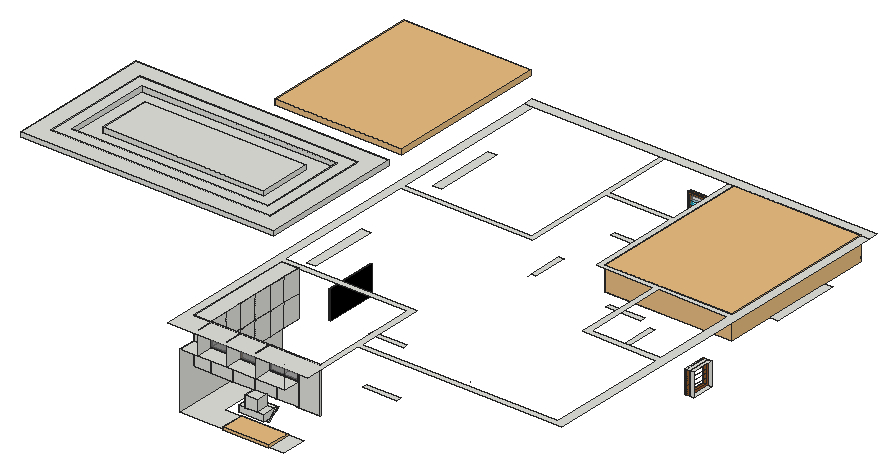
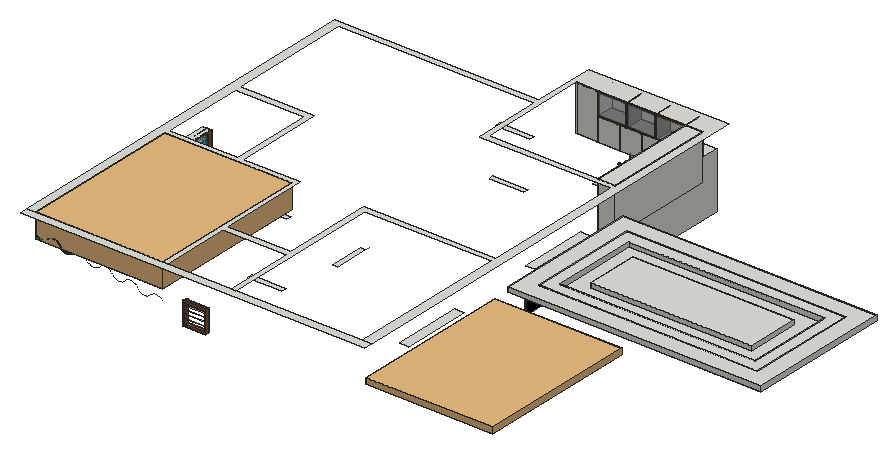
# SketchUp Ruby script. Lengths in inches.
U = 1.inch
M = Sketchup.active_model
def pt(a) = Geom::Point3d.new(a.map { |v| v * U })
def face(e, loops, mat)
  f = e.add_face(loops[0].map { |a| pt(a) })
  loops[1..].each { |l| e.add_face(l.map { |a| pt(a) }).erase! }
  f.material = f.back_material = mat if mat
  f
end
# faces: each face lists its corners as indices into pts; further lists are holes
def faces(e, pts, list, mat = nil) = list.each { |f| face(e, (f[0].is_a?(Array) ? f : [f]).map { |l| l.map { |i| pts[i] } }, mat) }
# xy, xz, yz: faces in a plane at the given z, y or x. An outline is a flat list of corners, or four numbers for a rectangle; further outlines are holes
def ring(l) = l.size == 4 ? [[l[0], l[1]], [l[2], l[1]], [l[2], l[3]], [l[0], l[3]]] : l.each_slice(2).to_a
def flat(e, list, mat, &to3) = list.each { |f| face(e, (f[0].is_a?(Array) ? f : [f]).map { |l| ring(l).map { |u, v| to3.(u, v) } }, mat) }
def xy(e, z, list, mat = nil) = flat(e, list, mat) { |x, y| [x, y, z] }
def xz(e, y, list, mat = nil) = flat(e, list, mat) { |x, z| [x, y, z] }
def yz(e, x, list, mat = nil) = flat(e, list, mat) { |y, z| [x, y, z] }
def lines(e, pts, list) = list.each { |a, b| e.add_line(pt(pts[a]), pt(pts[b])) }
# prism: a flat outline (further loops are holes) pulled along v
def prism(e, loops, v, mat = nil)
  f = face(e, loops, mat); d = Geom::Vector3d.new(v.map { |x| x * U })
  f.pushpull(f.normal.samedirection?(d) ? d.length : -d.length)
end
def box(e, o, s, mat = nil) = prism(e, [[o, [o[0] + s[0], o[1], o[2]], [o[0] + s[0], o[1] + s[1], o[2]], [o[0], o[1] + s[1], o[2]]]], [0, 0, s[2]], mat)
def at(x, y, z, deg = 0) = Geom::Transformation.translation(pt([x, y, z])) * Geom::Transformation.rotation(ORIGIN, Z_AXIS, deg.degrees)
def axes(o, x, y, z) = Geom::Transformation.new([*x, 0, *y, 0, *z, 0, *pt(o).to_a, 1])
def part(name) = M.definitions.add(name)
# library, detail: a bought-in or finely detailed component or shape, given as its bounding box
def library(name, o, s) = part(name).tap { |d| box(d.entities, o, s) }
def detail(e, o, s) = box(e.add_group.entities, o, s)
def put(e, d, t, mat = nil) = e.add_instance(d, t).tap { |i| i.material = mat if mat }
def group(e, t, mat = nil) = e.add_group.tap { |g| g.transformation = t; g.material = mat if mat }.entities
root = M.entities
M.materials.add("[Color C08]").color = [102, 51, 0]
M.materials.add("[Color_009]").color = [0, 0, 0]
M.materials.add("[Translucent Glass Gray]").color = [128, 128, 128]
M.materials["[Translucent Glass Gray]"].alpha = 0.5
M.materials.add("[Translucent Glass Tinted]1").color = [7, 201, 240]
M.materials["[Translucent Glass Tinted]1"].alpha = 0.48
M.materials.add("[Translucent_Glass_Gray]3").color = [128, 128, 128]
M.materials["[Translucent_Glass_Gray]3"].alpha = 0.5
M.materials.add("[Wood Cherry Original]").color = [152, 86, 42]
M.materials.add("[Wood Floor Parquet]").color = [145, 89, 39]
c1 = library("Gas cooktop",[0,0,34.52],[24.41,48.07,2.63])
c2 = part("Inclined chimney")
g1 = group(c2.entities,at(1.97,2.08,2.89))
xy(g1,0,[[0,7.9,31.3,13.68]])
xy(g1,11.29,[[0,0,31.3,13.68]])
xz(g1,13.68,[[0,0,31.3,11.29]])
yz(g1,0,[[7.9,0,0,11.29,13.68,11.29,13.68,0]])
yz(g1,31.3,[[7.9,0,13.68,0,13.68,11.29,0,11.29]])
g2 = group(c2.entities,at(0,9.85,0.4))
g3 = group(g2,at(0,0.61,0.43))
prism(g3,[[[35.24,0,0],[35.24,-3.39,4.84],[35.24,-3.58,4.7],[35.24,-0.29,0]]],[-35.24,0,0])
g4 = group(g2,at(0,-3.21,4.99))
prism(g4,[[[35.24,-0.2,-0.12],[35.24,-3.16,5],[0,-3.16,5],[0,-0.2,-0.12]]],[0,0.2,0.12])
g5 = group(g2,at(0,-6.27,10.27))
prism(g5,[[[35.24,-0.19,-0.14],[35.24,-3.58,4.7],[0,-3.58,4.7],[0,-0.19,-0.14]]],[0,0.19,0.14])
g6 = group(g2,at(0,0.61,0.43))
prism(g6,[[[35.24,0,0],[35.24,0.96,0],[35.24,-9.52,14.96],[35.24,-10.16,14.51]]],[-35.24,0,0])
g7 = group(c2.entities,at(10.24,3.95,20.8))
box(g7,[0,0,-6.62],[14.76,11.8125,20.56])
g8 = group(c2.entities,at(0,10.1,0))
prism(g8,[[[35.24,0.46,0],[35.24,1.33,0],[35.24,1.33,0.83],[35.24,1.01,0.83],[35.24,0.37,0.83],[35.24,0,0.83],[35.24,0,0.64]]],[-35.24,0,0])
c3 = part("Inclined+chimney")
put(c3.entities,c2,at(34.17,38.97,0.69))
c4 = part("ventilator")
g9 = group(c4.entities,at(0,0,0))
xy(g9,0,[[0,0,24,1],[0,1,24,6.83]],"[Wood Floor Parquet]")
xy(g9,1.75,[[2,0,22,6.83]],"[Wood Floor Parquet]")
xy(g9,21.87,[[2,0,22,6.83]],"[Wood Cherry Original]")
xy(g9,23.62,[[0,0,24,1],[0,1,24,6.83]],"[Wood Floor Parquet]")
xz(g9,0,[[[0,0,24,23.62],[2,1.75,22,21.87]]],"[Wood Floor Parquet]")
xz(g9,6.83,[[[0,0,24,23.62],[2,1.75,22,21.87]]],"[Wood Cherry Original]")
yz(g9,0,[[0,0,1,23.62],[1,0,6.83,23.62]],"[Wood Floor Parquet]")
yz(g9,2,[[0,1.75,6.83,1.75,6.83,7.66,0,3.5],[0,3.5,6.83,7.66,6.83,11.8125,0,7.66],[0,7.66,6.83,11.8125,6.83,15.97,0,11.8125],[0,11.8125,6.83,15.97,6.83,20.12,0,15.97],[0,15.97,6.83,20.12,6.83,21.87,0,21.87]],"[Wood Floor Parquet]")
yz(g9,22,[[0,1.75,0,3.5,6.83,7.66,6.83,1.75],[0,3.5,0,7.66,6.83,11.8125,6.83,7.66],[0,7.66,0,11.8125,6.83,15.97,6.83,11.8125],[0,11.8125,0,15.97,6.83,20.12,6.83,15.97],[0,15.97,0,21.87,6.83,21.87,6.83,20.12]],"[Wood Floor Parquet]")
yz(g9,24,[[0,0,1,23.62],[1,0,6.83,23.62]],"[Wood Floor Parquet]")
p = [[2,0,3.5],[2,6.83,7.66],[22,6.83,7.66],[22,0,3.5],[2,6.83,11.8125],[2,0,7.66],
  [22,0,7.66],[22,6.83,11.8125],[2,0,11.8125],[2,6.83,15.97],[22,6.83,15.97],[22,0,11.8125],
  [2,6.83,20.12],[2,0,15.97],[22,0,15.97],[22,6.83,20.12]]
faces(g9,p,[[0,1,2,3],[4,5,6,7],[8,9,10,11]],"[Translucent Glass Tinted]1")
faces(g9,p,[[12,13,14,15]],"[Translucent Glass Gray]")
c5 = library("Group\#27",[0,0,0],[132.5,168.5,25.21])
c6 = part("Component\#5")
box(c6.entities,[0,0,0],[30.3,0.18,23.6])
c7 = part("Group\#29")
xy(c7.entities,23.6,[[0,0.18,30.3,0.28]])
xz(c7.entities,0.28,[[[0,0,30.3,23.6],[1,1,29.3,22.6]]],"[Color C08]")
put(c7.entities,c6,at(0,0,0),"[Translucent_Glass_Gray]3")
c8 = library("Group\#16",[0,0,0],[132.5,168.5,6])
xy(root,37,[[301.397,9,409.897,9,409.897,35,327.397,35,327.397,141.5,301.397,141.5]])
xy(root,72,[[301.397,27,319.217,141.5],[643.397,241.399,652.397,265.051]])
xy(root,72.2,[[319.597,26.82,342.097,27],[342.497,26.82,364.997,27],[365.397,26.82,387.897,27],[388.297,26.82,410.797,27],[411.197,26.82,433.697,27],
  [319.217,27.2,319.397,45.883],[319.217,46.283,319.397,64.967],[319.217,65.367,319.397,84.05],[319.217,84.45,319.397,103.133],[319.217,103.533,319.397,122.217],
  [319.217,122.617,319.397,141.3]])
xy(root,84,[[443.897,69.5,479.897,74.5],[392.897,141.5,428.897,146.5],[565.897,256.5,570.897,292.5],[515.897,297.5,551.897,302.5],[433.897,302.5,438.897,338.5],
  [443.897,393.5,479.897,398.5]])
xy(root,92.408,[[610.289,470,610.297,471]])
xy(root,95.8,[[319.597,26.82,342.097,27],[342.497,26.82,364.997,27],[365.397,26.82,387.897,27],[388.297,26.82,410.797,27]])
xy(root,96,[[319.217,27.2,319.397,45.883],[319.217,46.283,319.397,64.967],[319.217,65.367,319.397,84.05],[319.217,84.45,319.397,103.133],[319.217,103.533,319.397,122.217],
  [319.217,122.617,319.397,141.3],[292.397,186,301.397,258],[643.397,241.399,652.397,265.051],[292.397,350.75,301.397,422.75],[643.397,350.75,652.397,422.75]])
xy(root,96.2,[[301.397,9,319.597,26.82],[319.597,9,349.897,26.82],[349.897,9,350.097,26.82],[350.097,9,380.297,26.82],[380.297,9,380.497,26.82],
  [380.497,9,410.797,26.82],[301.397,26.82,319.397,27],[380.497,27,410.797,27.1]])
xy(root,96.4,[[319.217,27.2,319.397,45.883],[319.217,46.283,319.397,64.967],[319.217,65.367,319.397,84.05],[319.217,84.45,319.397,103.133],[319.217,103.533,319.397,122.217],
  [319.217,122.617,319.397,141.3]])
xy(root,97.2,[[381.497,27,409.797,27.1]])
xy(root,101.49,[[624.897,470,624.899,471]])
xy(root,101.493,[[625.027,470,625.155,471]])
xy(root,118.8,[[381.497,27,409.797,27.1]])
xy(root,119.8,[[319.597,9,349.897,26.82],[350.097,9,380.297,26.82],[411.197,26.82,433.697,27],[319.597,27,349.897,27.1],[319.217,27.2,319.397,45.883],
  [319.217,46.283,319.397,64.967],[319.217,65.367,319.397,84.05],[319.217,84.45,319.397,103.133],[319.217,103.533,319.397,122.217],[319.217,122.617,319.397,141.3]])
xy(root,120,[[[292.397,3.625,438.897,3.625,438.897,69.5,652.397,69.5,652.397,471,643.397,471,643.397,302.5,510.897,302.5,510.897,471,505.897,471,505.897,398.5,438.897,398.5,438.897,471,433.897,471,433.897,302.5,301.397,302.5,301.397,471,292.397,471],[438.897,74.5,438.897,146.5,301.397,146.5,301.397,297.5,438.897,297.5,438.897,393.5,505.897,393.5,505.897,297.5,565.897,297.5,565.897,204,643.397,204,643.397,74.5],[301.397,26.82,433.897,141.5],[570.897,210,643.397,297.5]],[301.397,26.82,319.397,26.82,319.397,27,319.217,27,319.217,141.5,301.397,141.5],[292.397,471,652.397,480]])
xz(root,26.82,[[319.597,72.2,342.097,96.2],[342.497,72.2,364.997,95.8],[365.397,72.2,387.897,95.8],[388.297,72.2,410.797,96.2],[411.197,72.2,433.697,119.8],
  [319.597,95.8,319.597,96.2,319.397,96.2,319.397,120,410.797,120,410.797,119.8,380.497,119.8,380.497,96.2,380.297,96.2,380.297,119.8,350.097,119.8,350.097,96.2,349.897,96.2,349.897,119.8,319.597,119.8,319.597,96.2,342.097,96.2,342.097,95.8],[342.497,95.8,364.997,96.2],[365.397,95.8,387.897,96.2],[388.297,95.8,410.797,96.2],[301.397,96.2,319.397,120],
  [411.197,119.8,433.697,120]])
xz(root,27,[[301.397,72,319.217,96.2],[319.597,72.2,342.097,95.8],[342.497,72.2,364.997,95.8],[365.397,72.2,387.897,95.8],[388.297,72.2,410.797,95.8],
  [319.217,96.2,319.397,120],[[380.497,96.2,410.797,119.8],[381.497,97.2,409.797,118.8]]])
xz(root,27.1,[[[319.597,96.2,349.897,119.8],[320.597,97.2,348.897,118.8]]],"[Color C08]")
xz(root,27.2,[[319.217,72.2,319.397,96],[319.217,96.4,319.397,119.8]])
xz(root,45.883,[[319.217,72.2,319.397,96],[319.217,96.4,319.397,119.8]])
xz(root,46.283,[[319.217,72.2,319.397,96],[319.217,96.4,319.397,119.8]])
xz(root,64.967,[[319.217,72.2,319.397,96],[319.217,96.4,319.397,119.8]])
xz(root,65.367,[[319.217,72.2,319.397,96],[319.217,96.4,319.397,119.8]])
xz(root,84.05,[[319.217,72.2,319.397,96],[319.217,96.4,319.397,119.8]])
xz(root,84.45,[[319.217,72.2,319.397,96],[319.217,96.4,319.397,119.8]])
xz(root,103.133,[[319.217,72.2,319.397,96],[319.217,96.4,319.397,119.8]])
xz(root,103.533,[[319.217,72.2,319.397,96],[319.217,96.4,319.397,119.8]])
xz(root,122.217,[[319.217,72.2,319.397,96],[319.217,96.4,319.397,119.8]])
xz(root,122.617,[[319.217,72.2,319.397,96],[319.217,96.4,319.397,119.8]])
xz(root,141.3,[[319.217,72.2,319.397,96],[319.217,96.4,319.397,119.8]])
xz(root,141.5,[[301.397,72,319.217,120]])
xz(root,241.399,[[643.397,72,652.397,96]])
xz(root,265.051,[[643.397,72,652.397,96]])
xz(root,470,[[605.697,93.805,605.697,93.9375,605.497,93.9375,605.535,93.912,605.649,93.836]])
xz(root,471,[[642.897,98.449,642.932,98.48,643.033,98.572,643.132,98.666,643.23,98.761,643.327,98.858,643.397,98.932,643.397,120,642.897,120],[643.397,98.932,643.421,98.957,643.515,99.056,643.606,99.158,643.696,99.261,643.785,99.365,643.872,99.47,643.897,99.503,643.897,120,643.397,120]])
yz(root,301.397,[[9,37,141.5,37,141.5,72,27,72,27,96.2,9,96.2],[27,72,141.5,120],[26.82,96.2,27,120]])
yz(root,319.217,[[[27,72,141.5,120],[65.367,72.2,84.05,96],[103.533,72.2,122.217,96],[122.617,72.2,141.3,96],[27.2,72.2,45.883,96],[84.45,72.2,103.133,96],[46.283,72.2,64.967,96],[65.367,96.4,84.05,119.8],[103.533,96.4,122.217,119.8],[122.617,96.4,141.3,119.8],[46.283,96.4,64.967,119.8],[27.2,96.4,45.883,119.8],[84.45,96.4,103.133,119.8]]])
yz(root,319.397,[[27.2,72.2,45.883,96],[46.283,72.2,64.967,96],[65.367,72.2,84.05,96],[84.45,72.2,103.133,96],[103.533,72.2,122.217,96],
  [122.617,72.2,141.3,96],[26.82,96.2,27,120],[27.2,96.4,45.883,119.8],[46.283,96.4,64.967,119.8],[65.367,96.4,84.05,119.8],
  [84.45,96.4,103.133,119.8],[103.533,96.4,122.217,119.8],[122.617,96.4,141.3,119.8]])
yz(root,319.597,[[26.82,72.2,27,95.8],[9,96.2,26.82,119.8]])
yz(root,342.097,[[26.82,72.2,27,95.8]])
yz(root,342.497,[[26.82,72.2,27,95.8]])
yz(root,349.897,[[9,96.2,26.82,119.8]])
yz(root,350.097,[[9,96.2,26.82,119.8]])
yz(root,364.997,[[26.82,72.2,27,95.8]])
yz(root,365.397,[[26.82,72.2,27,95.8]])
yz(root,380.297,[[9,96.2,26.82,119.8]])
yz(root,380.497,[[9,96.2,26.82,119.8],[27,96.2,27.1,119.8]])
yz(root,381.497,[[27,97.2,27.1,118.8]])
yz(root,387.897,[[26.82,72.2,27,95.8]])
yz(root,388.297,[[26.82,72.2,27,95.8]])
yz(root,409.797,[[27,97.2,27.1,118.8]])
yz(root,410.797,[[26.82,72.2,27,95.8],[27,96.2,27.1,119.8]])
yz(root,411.197,[[26.82,72.2,27,96],[26.82,96,27,119.8]])
yz(root,433.697,[[26.82,72.2,27,119.8]])
p = [[609.471,470,92.46],[609.607,470,92.446],[609.607,471,92.446],[609.471,471,92.46],[609.743,470,92.434],[609.743,471,92.434],
  [609.879,470,92.425],[609.879,471,92.425],[610.016,470,92.417],[610.016,471,92.417],[610.152,470,92.411],[610.152,471,92.411],
  [610.289,470,92.408],[610.289,471,92.408],[610.497,470,92.407],[610.562,470,92.408],[610.562,471,92.408],[610.497,471,92.407],
  [610.699,470,92.411],[610.699,471,92.411],[610.835,470,92.416],[610.835,471,92.416],[610.972,470,92.423],[610.972,471,92.423],
  [611.108,470,92.433],[611.108,471,92.433],[611.244,470,92.444],[611.244,471,92.444],[611.38,470,92.458],[611.38,471,92.458],
  [608.795,470,92.5625],[608.93,470,92.538],[608.93,471,92.538],[608.795,471,92.5625],[609.065,470,92.515],[609.065,471,92.515],
  [609.097,470,92.51],[609.097,471,92.51],[609.335,470,92.477],[609.335,471,92.477],[609.297,470,92.482],[609.297,471,92.482],
  [611.497,470,92.472],[611.497,471,92.472],[611.697,470,92.498],[611.786,470,92.512],[611.786,471,92.512],[611.697,471,92.498],
  [611.921,470,92.534],[611.921,471,92.534],[612.056,470,92.558],[612.056,471,92.558],[608.262,470,92.682],[608.395,470,92.649],
  [608.395,471,92.649],[608.262,471,92.682],[608.528,470,92.618],[608.528,471,92.618],[608.661,470,92.589],[608.661,471,92.589],
  [612.19,470,92.584],[612.19,471,92.584],[612.323,470,92.613],[612.323,471,92.613],[612.457,470,92.643],[612.457,471,92.643],
  [612.589,470,92.676],[612.589,471,92.676],[608.13,470,92.717],[608.13,471,92.717],[608.097,470,92.726],[608.097,471,92.726],
  [612.697,470,92.705],[612.697,471,92.705],[607.608,470,92.878],[607.737,470,92.834],[607.737,471,92.834],[607.608,471,92.878],
  [607.868,470,92.793],[607.868,471,92.793],[607.897,470,92.784],[607.897,471,92.784],[612.897,470,92.761],[612.984,470,92.786],
  [612.984,471,92.786],[612.897,471,92.761],[613.114,470,92.827],[613.114,471,92.827],[613.244,470,92.87],[613.244,471,92.87],
  [607.351,470,92.97],[607.479,470,92.923],[607.479,471,92.923],[607.351,471,92.97],[613.373,470,92.915],[613.373,471,92.915],
  [613.502,470,92.962],[613.502,471,92.962],[607.097,470,93.071],[607.223,470,93.019],[607.223,471,93.019],[607.097,471,93.071],
  [613.629,470,93.011],[613.629,471,93.011],[613.756,470,93.062],[613.756,471,93.062],[606.897,470,93.156],[606.971,470,93.124],
  [606.971,471,93.124],[606.897,471,93.156],[613.882,470,93.115],[613.882,471,93.115],[613.897,470,93.122],[613.897,471,93.122],
  [606.598,470,93.295],[606.697,470,93.248],[606.697,471,93.248],[606.598,471,93.295],[614.097,470,93.211],[614.131,470,93.226],
  [614.131,471,93.226],[614.097,471,93.211],[614.255,470,93.285],[614.255,471,93.285],[606.476,470,93.356],[606.476,471,93.356],
  [614.377,470,93.346],[614.377,471,93.346],[614.499,470,93.408],[614.499,471,93.408],[606.235,470,93.484],[606.355,470,93.419],
  [606.355,471,93.419],[606.235,471,93.484],[614.619,470,93.473],[614.619,471,93.473],[606.115,470,93.551],[606.115,471,93.551],
  [614.739,470,93.539],[614.739,471,93.539],[614.857,470,93.608],[614.857,471,93.608],[605.88,470,93.69],[605.997,470,93.619],
  [605.997,471,93.619],[605.88,471,93.69],[614.974,470,93.678],[614.974,471,93.678],[605.764,470,93.762],[605.764,471,93.762],
  [615.09,470,93.749],[615.09,471,93.749],[615.097,470,93.754],[615.097,471,93.754],[605.697,470,93.805],[605.697,471,93.805],
  [615.297,470,93.884],[615.319,470,93.899],[615.319,471,93.899],[615.297,471,93.884],[615.432,470,93.976],[615.432,471,93.976],
  [615.544,470,94.055],[615.544,471,94.055],[615.654,470,94.136],[615.654,471,94.136],[615.763,470,94.218],[615.763,471,94.218],
  [615.87,470,94.302],[615.87,471,94.302],[615.977,470,94.388],[615.977,471,94.388],[616.082,470,94.476],[616.082,471,94.476],
  [616.185,470,94.565],[616.185,471,94.565],[616.288,470,94.655],[616.288,471,94.655],[616.297,470,94.664],[616.297,471,94.664],
  [616.497,470,94.851],[616.585,470,94.937],[616.585,471,94.937],[616.497,471,94.851],[616.682,470,95.034],[616.682,471,95.034],
  [616.777,470,95.132],[616.777,471,95.132],[616.87,470,95.232],[616.87,471,95.232],[616.961,470,95.334],[616.961,471,95.334],
  [617.051,470,95.436],[617.051,471,95.436],[617.14,470,95.54],[617.14,471,95.54],[617.227,470,95.646],[617.227,471,95.646],
  [617.312,470,95.753],[617.312,471,95.753],[617.395,470,95.861],[617.395,471,95.861],[617.477,470,95.971],[617.477,471,95.971],
  [617.497,470,96.031],[617.497,471,96.031],[636.388,470,96.259],[636.524,470,96.249],[636.524,471,96.249],[636.388,471,96.259],
  [636.661,470,96.241],[636.661,471,96.241],[636.697,470,96.24],[636.697,471,96.24],[636.934,470,96.232],[637.07,470,96.231],
  [637.07,471,96.231],[636.934,471,96.232],[636.897,470,96.233],[636.897,471,96.233],[637.207,470,96.232],[637.207,471,96.232],
  [637.344,470,96.235],[637.344,471,96.235],[637.48,470,96.24],[637.48,471,96.24],[637.617,470,96.247],[637.617,471,96.247],
  [637.753,470,96.257],[637.753,471,96.257],[635.71,470,96.34],[635.845,470,96.319],[635.845,471,96.319],[635.71,471,96.34],
  [635.697,470,96.342],[635.697,471,96.342],[635.98,470,96.301],[635.98,471,96.301],[636.116,470,96.285],[636.116,471,96.285],
  [636.252,470,96.271],[636.252,471,96.271],[637.889,470,96.268],[637.889,471,96.268],[637.897,470,96.269],[637.897,471,96.269],
  [638.097,470,96.291],[638.161,470,96.298],[638.161,471,96.298],[638.097,471,96.291],[638.296,470,96.316],[638.296,471,96.316],
  [638.431,470,96.336],[638.431,471,96.336],[638.566,470,96.358],[638.566,471,96.358],[635.04,470,96.473],[635.173,470,96.442],
  [635.173,471,96.442],[635.04,471,96.473],[635.306,470,96.413],[635.306,471,96.413],[635.44,470,96.387],[635.44,471,96.387],
  [635.497,470,96.376],[635.497,471,96.376],[638.701,470,96.382],[638.701,471,96.382],[638.835,470,96.409],[638.835,471,96.409],
  [638.968,470,96.437],[638.968,471,96.437],[639.097,470,96.467],[639.097,471,96.467],[634.644,470,96.578],[634.775,470,96.541],
  [634.775,471,96.541],[634.644,471,96.578],[634.907,470,96.506],[634.907,471,96.506],[639.297,470,96.517],[639.366,470,96.535],
  [639.366,471,96.535],[639.297,471,96.517],[639.498,470,96.572],[639.498,471,96.572],[617.697,470,96.561],[617.701,470,96.57],
  [617.701,471,96.57],[617.697,471,96.561],[617.752,470,96.6875],[617.752,471,96.6875],[634.513,470,96.617],[634.513,471,96.617],
  [634.497,470,96.622],[634.497,471,96.622],[639.629,470,96.611],[639.629,471,96.611],[639.759,470,96.652],[639.759,471,96.652],
  [617.804,470,96.804],[617.804,471,96.804],[633.996,470,96.794],[634.124,470,96.747],[634.124,471,96.747],[633.996,471,96.794],
  [634.253,470,96.702],[634.253,471,96.702],[634.297,470,96.687],[634.297,471,96.687],[639.889,470,96.694],[639.889,471,96.694],
  [640.018,470,96.739],[640.018,471,96.739],[640.146,470,96.786],[640.146,471,96.786],[617.858,470,96.92],[617.858,471,96.92],
  [633.741,470,96.895],[633.868,470,96.844],[633.868,471,96.844],[633.741,471,96.895],[640.274,470,96.835],[640.274,471,96.835],
  [640.297,470,96.845],[640.297,471,96.845],[617.914,470,97.035],[617.914,471,97.035],[633.491,470,97.003],[633.616,470,96.948],
  [633.616,471,96.948],[633.491,471,97.003],[640.497,470,96.927],[640.527,470,96.939],[640.527,471,96.939],[640.497,471,96.927],
  [640.652,470,96.994],[640.652,471,96.994],[617.972,470,97.149],[617.972,471,97.149],[633.367,470,97.061],[633.367,471,97.061],
  [640.776,470,97.051],[640.776,471,97.051],[618.032,470,97.262],[618.032,471,97.262],[633.297,470,97.094],[633.297,471,97.094],
  [640.9,470,97.109],[640.9,471,97.109],[641.022,470,97.17],[641.022,471,97.17],[632.879,470,97.308],[633,470,97.243],
  [633,471,97.243],[632.879,471,97.308],[633.097,470,97.193],[633.097,471,97.193],[641.144,470,97.233],[641.144,471,97.233],
  [641.264,470,97.297],[641.264,471,97.297],[618.094,470,97.375],[618.094,471,97.375],[632.76,470,97.375],[632.76,471,97.375],
  [641.383,470,97.364],[641.383,471,97.364],[618.157,470,97.486],[618.157,471,97.486],[632.525,470,97.514],[632.642,470,97.443],
  [632.642,471,97.443],[632.525,471,97.514],[641.497,470,97.429],[641.497,471,97.429],[618.222,470,97.596],[618.222,471,97.596],
  [632.409,470,97.586],[632.409,471,97.586],[618.289,470,97.705],[618.289,471,97.705],[632.294,470,97.66],[632.294,471,97.66],
  [641.697,470,97.55],[641.735,470,97.574],[641.735,471,97.574],[641.697,471,97.55],[641.85,470,97.647],[641.85,471,97.647],
  [641.964,470,97.723],[641.964,471,97.723],[618.357,470,97.813],[618.357,471,97.813],[632.097,470,97.793],[632.18,470,97.736],
  [632.18,471,97.736],[632.097,471,97.793],[642.077,470,97.8],[642.077,471,97.8],[618.428,470,97.92],[618.428,471,97.92],
  [642.189,470,97.879],[642.189,471,97.879],[618.499,470,98.026],[618.499,471,98.026],[631.846,470,97.974],[631.897,470,97.936],
  [631.897,471,97.936],[631.846,471,97.974],[642.299,470,97.96],[642.299,471,97.96],[618.573,470,98.131],[618.573,471,98.131],
  [631.738,470,98.056],[631.738,471,98.056],[642.408,470,98.042],[642.408,471,98.042],[642.515,470,98.126],[642.515,471,98.126],
  [618.648,470,98.234],[618.648,471,98.234],[631.524,470,98.227],[631.63,470,98.141],[631.63,471,98.141],[631.524,471,98.227],
  [642.622,470,98.212],[642.622,471,98.212],[618.697,470,98.3],[618.697,471,98.3],[631.419,470,98.315],[631.419,471,98.315],
  [642.697,470,98.275],[642.697,471,98.275],[631.316,470,98.404],[631.316,471,98.404],[631.214,470,98.495],[631.214,471,98.495],
  [642.897,470,98.449],[642.932,470,98.48],[642.932,471,98.48],[642.897,471,98.449],[631.114,470,98.588],[631.114,471,98.588],
  [643.033,470,98.572],[643.033,471,98.572],[618.897,470,98.554],[618.966,470,98.636],[618.966,471,98.636],[618.897,471,98.554],
  [619.049,470,98.733],[619.049,471,98.733],[631.015,470,98.682],[631.015,471,98.682],[643.132,470,98.666],[643.132,471,98.666],
  [619.134,470,98.829],[619.134,471,98.829],[630.917,470,98.777],[630.917,471,98.777],[643.23,470,98.761],[643.23,471,98.761],
  [619.22,470,98.924],[619.22,471,98.924],[630.897,470,98.797],[630.897,471,98.797],[643.327,470,98.858],[643.327,471,98.858],
  [619.308,470,99.017],[619.308,471,99.017],[643.421,470,98.957],[643.421,471,98.957],[643.397,471,98.932],[619.397,470,99.108],
  [619.397,471,99.108],[630.633,470,99.073],[630.697,470,99.004],[630.697,471,99.004],[630.633,471,99.073],[643.515,470,99.056],
  [643.515,471,99.056],[619.488,470,99.199],[619.488,471,99.199],[630.542,470,99.175],[630.542,471,99.175],[643.606,470,99.158],
  [643.606,471,99.158],[619.58,470,99.288],[619.58,471,99.288],[630.452,470,99.278],[630.452,471,99.278],[643.696,470,99.261],
  [643.696,471,99.261],[619.674,470,99.375],[619.674,471,99.375],[630.364,470,99.382],[630.364,471,99.382],[643.785,470,99.365],
  [643.785,471,99.365],[619.769,470,99.461],[619.769,471,99.461],[630.278,470,99.488],[630.278,471,99.488],[643.872,470,99.47],
  [643.872,471,99.47],[619.865,470,99.545],[619.865,471,99.545],[619.897,470,99.573],[619.897,471,99.573],[630.193,470,99.595],
  [630.193,471,99.595],[643.897,470,99.503],[643.897,471,99.503],[630.11,470,99.704],[630.11,471,99.704],[620.097,470,99.738],
  [620.162,470,99.789],[620.162,471,99.789],[620.097,471,99.738],[630.028,470,99.813],[630.028,471,99.813],[620.263,470,99.867],
  [620.263,471,99.867],[629.926,470,99.891],[629.926,471,99.891],[620.366,470,99.943],[620.366,471,99.943],[620.47,470,100.018],
  [620.47,471,100.018],[629.823,470,99.967],[629.823,471,99.967],[620.575,470,100.091],[620.575,471,100.091],[629.719,470,100.041],
  [629.719,471,100.041],[629.697,470,100.056],[629.697,471,100.056],[620.681,470,100.162],[620.681,471,100.162],[620.788,470,100.232],
  [620.788,471,100.232],[620.897,470,100.3],[620.897,471,100.3],[629.399,470,100.254],[629.497,470,100.19],[629.497,471,100.19],
  [629.399,471,100.254],[621.006,470,100.366],[621.006,471,100.366],[629.18,470,100.387],[629.29,470,100.321],[629.29,471,100.321],
  [629.18,471,100.387],[621.097,470,100.419],[621.097,471,100.419],[629.07,470,100.451],[629.07,471,100.451],[621.297,470,100.531],
  [621.341,470,100.554],[621.341,471,100.554],[621.297,471,100.531],[628.845,470,100.573],[628.958,470,100.513],[628.958,471,100.513],
  [628.845,471,100.573],[621.454,470,100.613],[621.454,471,100.613],[621.569,470,100.671],[621.569,471,100.671],[628.616,470,100.688],
  [628.731,470,100.632],[628.731,471,100.632],[628.616,471,100.688],[621.684,470,100.726],[621.684,471,100.726],[621.8,470,100.78],
  [621.8,471,100.78],[628.501,470,100.743],[628.501,471,100.743],[628.497,470,100.745],[628.497,471,100.745],[621.917,470,100.832],
  [621.917,471,100.832],[622.035,470,100.882],[622.035,471,100.882],[628.149,470,100.897],[628.267,470,100.848],[628.267,471,100.848],
  [628.149,471,100.897],[628.297,470,100.834],[628.297,471,100.834],[622.154,470,100.93],[622.154,471,100.93],[622.273,470,100.976],
  [622.273,471,100.976],[627.91,470,100.99],[628.03,470,100.944],[628.03,471,100.944],[627.91,471,100.99],[622.297,470,100.985],
  [622.297,471,100.985],[627.669,470,101.075],[627.79,470,101.033],[627.79,471,101.033],[627.669,471,101.075],[622.497,470,101.056],
  [622.514,470,101.062],[622.514,471,101.062],[622.497,471,101.056],[622.636,470,101.103],[622.636,471,101.103],[622.758,470,101.141],
  [622.758,471,101.141],[622.88,470,101.178],[622.88,471,101.178],[627.425,470,101.153],[627.547,470,101.115],[627.547,471,101.115],
  [627.425,471,101.153],[623.004,470,101.212],[623.004,471,101.212],[623.127,470,101.245],[623.127,471,101.245],[623.252,470,101.275],
  [623.252,471,101.275],[627.055,470,101.255],[627.097,470,101.244],[627.097,471,101.244],[627.055,471,101.255],[627.302,470,101.189],
  [627.302,471,101.189],[627.297,470,101.19],[627.297,471,101.19],[623.376,470,101.304],[623.376,471,101.304],[623.497,470,101.33],
  [623.497,471,101.33],[626.555,470,101.362],[626.68,470,101.338],[626.68,471,101.338],[626.555,471,101.362],[626.806,470,101.3125],
  [626.806,471,101.3125],[626.93,470,101.284],[626.93,471,101.284],[623.697,470,101.368],[623.753,470,101.378],[623.753,471,101.378],
  [623.697,471,101.368],[623.88,470,101.398],[623.88,471,101.398],[624.006,470,101.417],[624.006,471,101.417],[624.133,470,101.434],
  [624.133,471,101.434],[624.26,470,101.448],[624.26,471,101.448],[624.388,470,101.461],[624.388,471,101.461],[626.097,470,101.432],
  [626.175,470,101.422],[626.175,471,101.422],[626.097,471,101.432],[626.302,470,101.404],[626.302,471,101.404],[626.428,470,101.384],
  [626.428,471,101.384],[624.515,470,101.471],[624.515,471,101.471],[624.643,470,101.48],[624.643,471,101.48],[624.697,470,101.482],
  [624.697,471,101.482],[624.899,470,101.49],[625.027,470,101.493],[625.027,471,101.493],[624.899,471,101.49],[625.155,470,101.493],
  [625.283,470,101.491],[625.283,471,101.491],[625.155,471,101.493],[625.41,470,101.488],[625.41,471,101.488],[625.538,470,101.482],
  [625.538,471,101.482],[625.666,470,101.474],[625.666,471,101.474],[625.794,470,101.464],[625.794,471,101.464],[625.897,470,101.454],
  [625.897,471,101.454],[301.397,777.071,120],[301.397,777.071,119],[523.962,470,83.878],[524.054,470,83.776],[524.097,470,83.729],
  [525.158,470,82.759],[525.267,470,82.677],[525.297,470,82.654],[526.3,470,82.011],[526.42,470,81.946],[526.497,470,81.906],
  [527.544,470,81.45],[527.673,470,81.405],[527.697,470,81.397],[528.727,470,81.116],[528.861,470,81.09],[528.897,470,81.083],
  [529.945,470,80.952],[530.081,470,80.944],[530.097,470,80.944],[531.173,470,80.96],[531.297,470,80.97],[532.389,470,81.14],
  [532.497,470,81.165],[533.567,470,81.489],[533.694,470,81.538],[533.697,470,81.539],[534.804,470,82.067],[534.897,470,82.12],
  [535.936,470,82.829],[536.042,470,82.915],[536.097,470,82.961],[537.117,470,83.964],[537.205,470,84.068],[537.292,470,84.173],
  [537.297,470,84.18],[511.92,470,82.729],[511.994,470,82.834],[512.069,470,82.9375],[512.097,470,82.976],[513.189,470,84.164],
  [513.285,470,84.248],[513.297,470,84.258],[514.317,470,85.003],[514.427,470,85.069],[514.497,470,85.11],[515.574,470,85.633],
  [515.694,470,85.679],[515.697,470,85.68],[516.797,470,86.007],[516.897,470,86.028],[517.936,470,86.174],[518.063,470,86.183],
  [518.097,470,86.184],[519.214,470,86.167],[519.297,470,86.159],[520.351,470,85.987],[520.475,470,85.957],[520.497,470,85.952],
  [521.569,470,85.6],[521.6875,470,85.551],[521.697,470,85.546],[522.711,470,85.024],[522.82,470,84.957],[522.897,470,84.906],
  [550.343,470,88.015],[550.429,470,87.91],[551.696,470,86.668],[551.697,470,86.667],[550.497,470,87.829],[555.238,470,84.969],
  [555.297,470,84.957],[551.589,470,86.754],[552.707,470,85.971],[552.825,470,85.902],[552.897,470,85.862],[553.933,470,85.371],
  [554.061,470,85.322],[555.105,470,85],[554.097,470,85.308],[556.453,470,84.786],[556.497,470,84.783],[557.682,470,84.775],
  [557.697,470,84.776],[559.954,470,85.222],[560.083,470,85.267],[562.473,470,86.57],[562.497,470,86.589],[556.317,470,84.798],
  [561.209,470,85.76],[561.297,470,85.807],[560.097,470,85.272],[563.672,470,87.685],[563.697,470,87.715],[563.58,470,87.584],
  [558.766,470,84.91],[558.897,470,84.935],[557.545,470,84.767],[562.364,470,86.487],[538.493,470,86.448],[538.497,470,86.454],
  [540.746,470,88.689],[540.854,470,88.759],[538.354,470,86.233],[538.423,470,86.341],[539.645,470,87.815],[539.697,470,87.863],
  [539.553,470,87.726],[545.604,470,90.009],[545.697,470,90.003],[540.897,470,88.787],[549.135,470,88.978],[549.246,470,88.914],
  [544.326,470,89.975],[544.453,470,89.988],[549.297,470,88.883],[541.983,470,89.359],[542.097,470,89.407],[544.497,470,89.992],
  [547.976,470,89.517],[548.095,470,89.472],[546.871,470,89.84],[546.897,470,89.834],[548.097,470,89.471],[546.746,470,89.866],
  [543.193,470,89.772],[543.297,470,89.798],[581.617,470,88.858],[581.697,470,88.838],[580.452,470,89.246],[580.497,470,89.228],
  [576.82,470,92.055],[576.897,470,91.954],[578.026,470,90.756],[578.097,470,90.694],[580.326,470,89.3],[584.054,470,88.586],
  [584.097,470,88.588],[582.826,470,88.636],[582.897,470,88.629],[576.738,470,92.165],[579.235,470,89.865],[579.297,470,89.828],
  [579.119,470,89.9375],[577.924,470,90.847],[589.941,470,91.113],[590.037,470,91.21],[588.787,470,90.152],[588.897,470,90.23],
  [564.804,470,89.726],[564.867,470,89.837],[587.61,470,89.461],[587.697,470,89.504],[585.142,470,88.6875],[585.276,470,88.71],
  [585.297,470,88.713],[583.917,470,88.583],[586.339,470,88.962],[586.47,470,89.003],[586.497,470,89.012],[590.097,470,91.273],
  [564.897,470,89.889],[570.843,470,93.785],[570.897,470,93.791],[567.18,470,92.369],[567.285,470,92.442],[567.297,470,92.451],
  [564.742,470,89.614],[566.018,470,91.368],[566.097,470,91.45],[568.394,470,93.078],[568.497,470,93.125],[575.555,470,92.925],
  [575.668,470,92.864],[565.93,470,91.275],[573.265,470,93.714],[573.297,470,93.708],[569.591,470,93.529],[569.697,470,93.559],
  [570.716,470,93.768],[575.697,470,92.848],[571.993,470,93.843],[572.097,470,93.84],[574.379,470,93.427],[574.497,470,93.386],
  [573.139,470,93.736],[607.999,470,92.754],[604.37,470,94.858],[604.469,470,94.763],[606.722,470,93.236],[606.846,470,93.179],
  [604.497,470,94.737],[612.721,470,92.711],[612.853,470,92.748],[611.651,470,92.492],[615.206,470,93.823],[614.007,470,93.17],
  [609.2,470,92.495],[616.488,470,94.842],[610.425,470,92.407],[616.388,470,94.748],[611.516,470,92.474],[591.27,470,93.211],
  [591.297,470,93.266],[599.657,470,97.58],[599.697,470,97.574],[592.489,470,95.005],[592.497,470,95.014],[593.517,470,95.964],
  [593.618,470,96.042],[594.81,470,96.789],[594.897,470,96.833],[602.086,470,96.807],[602.097,470,96.802],[591.214,470,93.096],
  [591.107,470,92.863],[591.159,470,92.98],[593.697,470,96.101],[597.108,470,97.553],[597.235,470,97.574],[592.321,470,94.812],
  [592.404,470,94.909],[597.297,470,97.583],[601.971,470,96.864],[603.281,470,96.067],[603.297,470,96.054],[599.53,470,97.598],
  [603.178,470,96.143],[598.382,470,97.669],[598.497,470,97.669],[600.78,470,97.329],[600.897,470,97.292],[595.991,470,97.278],
  [596.097,470,97.312],[634.382,470,96.659],[641.619,470,97.502],[633.121,470,97.181],[633.243,470,97.12],[630.821,470,98.875],
  [632.068,470,97.813],[635.575,470,96.362],[642.727,470,98.3],[642.83,470,98.389],[636.797,470,96.236],[631.956,470,97.893],
  [640.401,470,96.886],[630.726,470,98.973],[641.502,470,97.432],[639.101,470,96.468],[639.234,470,96.5],[625.921,470,101.452],
  [626.048,470,101.438],[617.518,470,96.092],[617.561,470,96.212],[638.025,470,96.282],[617.653,470,96.451],[620.061,470,99.709],
  [622.393,470,101.02],[617.606,470,96.332],[627.179,470,101.223],[643.957,470,99.577],[644.04,470,99.685],[618.804,470,98.438],
  [618.884,470,98.538],[644.122,470,99.795],[618.725,470,98.337],[624.771,470,101.486],[624.897,470,101.49],[623.627,470,101.355],
  [629.613,470,100.114],[619.962,470,99.628],[621.228,470,100.493],[629.507,470,100.184],[628.384,470,100.796],[621.117,470,100.431],
  [623.502,470,101.33],[534.697,470,82.007],[527.497,470,81.467],[511.897,470,82.696],[533.497,470,81.464],[537.097,470,83.942],
  [535.897,470,82.8],[531.097,470,80.955],[532.297,470,81.121],[513.097,470,84.081],[515.497,470,85.601],[514.297,470,84.991],
  [516.697,470,85.984],[521.497,470,85.629],[519.097,470,86.176],[517.897,470,86.171],[520.297,470,85.999],[528.697,470,81.123],
  [522.697,470,85.032],[523.897,470,83.953],[525.097,470,82.807],[526.297,470,82.013],[529.897,470,80.955],[545.497,470,90.014],
  [569.497,470,93.501],[579.097,470,89.951],[546.697,470,89.875],[557.497,470,84.766],[561.097,470,85.703],[587.497,470,89.407],
  [588.697,470,90.09],[591.097,470,92.841],[589.897,470,91.071],[551.497,470,86.831],[565.897,470,91.239],[559.897,470,85.203],
  [550.297,470,88.073],[593.497,470,95.949],[594.697,470,96.731],[595.897,470,97.247],[597.097,470,97.552],[549.097,470,88.999],
  [552.697,470,85.977],[563.497,470,87.495],[564.697,470,89.529],[567.097,470,92.31],[571.897,470,93.844],[544.297,470,89.972],
  [541.897,470,89.321],[553.897,470,85.385],[573.097,470,93.742],[540.697,470,88.657],[577.897,470,90.871],[547.897,470,89.545],
  [555.097,470,85.002],[575.497,470,92.954],[581.497,470,88.889],[580.297,470,89.312],[562.297,470,86.438],[538.297,470,86.14],
  [556.297,470,84.8],[539.497,470,87.671],[576.697,470,92.196],[592.297,470,94.784],[570.697,470,93.766],[574.297,470,93.453],
  [568.297,470,93.031],[558.697,470,84.897],[582.697,470,88.651],[583.897,470,88.583],[586.297,470,88.95],[585.097,470,88.681],
  [543.097,470,89.747],[433.897,297.5,84],[433.897,302.5,84],[600.697,470,97.353],[604.297,470,94.928],[599.497,470,97.602],
  [601.897,470,96.899],[603.097,470,96.2],[610.297,470,92.408],[598.297,470,97.667],[1014.718,-502.818,541.354],[1014.716,-502.818,541.354],
  [1014.716,-502.818,540.318],[1014.718,-502.818,540.318],[438.897,338.5,84],[438.897,338.815,84],[410.797,9,120],[410.797,9,96.2],
  [380.497,27,119.8],[410.797,26.82,119.8],[410.797,26.82,96.2]]
faces(root,p,[[0,1,2,3],[1,4,5,2],[4,6,7,5],[6,8,9,7],[8,10,11,9],[10,12,13,11],[14,15,16,17],[15,18,19,16],
  [18,20,21,19],[20,22,23,21],[22,24,25,23],[24,26,27,25],[26,28,29,27],[30,31,32,33],[31,34,35,32],[34,36,37,35],
  [38,0,3,39],[40,38,39,41],[28,42,43,29],[44,45,46,47],[45,48,49,46],[48,50,51,49],[52,53,54,55],[53,56,57,54],
  [56,58,59,57],[58,30,33,59],[50,60,61,51],[60,62,63,61],[62,64,65,63],[64,66,67,65],[68,52,55,69],[70,68,69,71],
  [66,72,73,67],[74,75,76,77],[75,78,79,76],[78,80,81,79],[82,83,84,85],[83,86,87,84],[86,88,89,87],[90,91,92,93],
  [91,74,77,92],[88,94,95,89],[94,96,97,95],[98,99,100,101],[99,90,93,100],[96,102,103,97],[102,104,105,103],[106,107,108,109],
  [107,98,101,108],[104,110,111,105],[110,112,113,111],[114,115,116,117],[118,119,120,121],[119,122,123,120],[124,114,117,125],[122,126,127,123],
  [126,128,129,127],[130,131,132,133],[131,124,125,132],[128,134,135,129],[136,130,133,137],[134,138,139,135],[138,140,141,139],[142,143,144,145],
  [143,136,137,144],[140,146,147,141],[148,142,145,149],[146,150,151,147],[150,152,153,151],[154,148,149,155],[156,157,158,159],[157,160,161,158],
  [160,162,163,161],[162,164,165,163],[164,166,167,165],[166,168,169,167],[168,170,171,169],[170,172,173,171],[172,174,175,173],[174,176,177,175],
  [176,178,179,177],[180,181,182,183],[181,184,185,182],[184,186,187,185],[186,188,189,187],[188,190,191,189],[190,192,193,191],[192,194,195,193],
  [194,196,197,195],[196,198,199,197],[198,200,201,199],[200,202,203,201],[202,204,205,203],[206,207,208,209],[207,210,211,208],[210,212,213,211],
  [214,215,216,217],[218,214,217,219],[215,220,221,216],[220,222,223,221],[222,224,225,223],[224,226,227,225],[226,228,229,227],[230,231,232,233],
  [234,230,233,235],[231,236,237,232],[236,238,239,237],[238,240,241,239],[240,206,209,241],[228,242,243,229],[242,244,245,243],[246,247,248,249],
  [247,250,251,248],[250,252,253,251],[252,254,255,253],[256,257,258,259],[257,260,261,258],[260,262,263,261],[262,264,265,263],[254,266,267,255],
  [266,268,269,267],[268,270,271,269],[270,272,273,271],[274,275,276,277],[275,278,279,276],[278,256,259,279],[280,281,282,283],[281,284,285,282],
  [286,287,288,289],[287,290,291,288],[292,274,277,293],[294,292,293,295],[284,296,297,285],[296,298,299,297],[290,300,301,291],[302,303,304,305],
  [303,306,307,304],[306,308,309,307],[298,310,311,299],[310,312,313,311],[312,314,315,313],[300,316,317,301],[318,319,320,321],[319,302,305,320],
  [314,322,323,315],[322,324,325,323],[316,326,327,317],[328,329,330,331],[329,318,321,330],[332,333,334,335],[333,336,337,334],[326,338,339,327],
  [340,328,331,341],[336,342,343,337],[338,344,345,339],[346,340,341,347],[342,348,349,343],[348,350,351,349],[352,353,354,355],[353,356,357,354],
  [350,358,359,351],[358,360,361,359],[344,362,363,345],[364,352,355,365],[360,366,367,361],[362,368,369,363],[370,371,372,373],[371,364,365,372],
  [366,374,375,367],[368,376,377,369],[378,370,373,379],[376,380,381,377],[382,378,379,383],[384,385,386,387],[385,388,389,386],[388,390,391,389],
  [380,392,393,381],[394,395,396,397],[395,382,383,396],[390,398,399,391],[392,400,401,393],[398,402,403,399],[400,404,405,401],[406,407,408,409],
  [402,410,411,403],[404,412,413,405],[414,406,409,415],[410,416,417,411],[416,418,419,417],[412,420,421,413],[422,423,424,425],[423,414,415,424],
  [418,426,427,419],[420,428,429,421],[430,422,425,431],[426,432,433,427],[434,430,431,435],[436,434,435,437],[438,439,440,441],[442,436,437,443],
  [439,444,445,440],[446,447,448,449],[447,450,451,448],[452,442,443,453],[444,454,455,445],[450,456,457,451],[458,452,453,459],[454,460,461,455],
  [456,462,463,457],[464,458,459,465],[460,466,467,461],[462,468,469,463],[466,470,471,472,467],[468,473,474,469],[475,476,477,478],[470,479,480,471],
  [473,481,482,474],[483,475,478,484],[479,485,486,480],[481,487,488,482],[489,483,484,490],[485,491,492,486],[487,493,494,488],[495,489,490,496],
  [491,497,498,492],[493,499,500,494],[501,495,496,502],[497,503,504,498],[499,505,506,500],[505,507,508,506],[509,501,502,510],[503,511,512,504],
  [513,509,510,514],[515,516,517,518],[519,513,514,520],[516,521,522,517],[523,519,520,524],[521,525,526,522],[525,527,528,526],[529,523,524,530],
  [527,531,532,528],[533,529,530,534],[535,533,534,536],[531,537,538,532],[537,539,540,538],[539,541,542,540],[543,544,545,546],[541,547,548,542],
  [549,550,551,552],[550,543,546,551],[547,553,554,548],[555,549,552,556],[557,558,559,560],[561,562,563,564],[562,555,556,563],[558,565,566,559],
  [565,567,568,566],[569,570,571,572],[570,561,564,571],[567,573,574,568],[573,575,576,574],[577,569,572,578],[579,577,578,580],[575,581,582,576],
  [581,583,584,582],[585,586,587,588],[586,589,590,587],[583,591,592,584],[591,593,594,592],[595,596,597,598],[596,585,588,597],[593,599,600,594],
  [601,602,603,604],[602,595,598,603],[605,606,607,608],[606,609,610,607],[609,611,612,610],[611,613,614,612],[615,616,617,618],[616,601,604,617],
  [613,619,620,614],[619,621,622,620],[621,623,624,622],[625,626,627,628],[629,615,618,630],[631,629,630,632],[623,633,634,624],[633,635,636,634],
  [637,638,639,640],[638,641,642,639],[641,643,644,642],[643,625,628,644],[645,646,647,648],[646,649,650,647],[649,651,652,650],[651,653,654,652],
  [653,655,656,654],[655,657,658,656],[659,660,661,662],[660,663,664,661],[663,665,666,664],[665,637,640,666],[657,667,668,658],[667,669,670,668],
  [669,671,672,670],[673,674,675,676],[677,678,679,680],[678,681,682,679],[681,683,684,682],[683,685,686,684],[685,687,688,686],[687,689,690,688]])
lines(root,p,[[691,692],[693,694],[694,695],[696,697],[697,698],[699,700],[700,701],[702,703],[703,704],[705,706],[706,707],[708,709],
  [709,710],[711,712],[713,714],[715,716],[716,717],[718,719],[720,721],[721,722],[723,724],[724,725],[725,726],[727,728],
  [728,729],[729,730],[731,732],[732,733],[734,735],[735,736],[737,738],[738,739],[740,741],[742,743],[743,744],[745,746],
  [747,748],[748,749],[750,751],[751,752],[753,754],[754,755],[756,757],[758,759],[757,760],[761,762],[763,758],[764,765],
  [765,766],[767,768],[769,761],[768,770],[771,772],[773,774],[775,776],[777,778],[779,771],[780,781],[776,782],[783,784],
  [785,783],[786,787],[788,773],[789,777],[790,791],[792,793],[794,795],[796,797],[795,790],[798,796],[799,800],[793,801],
  [802,803],[804,805],[803,806],[807,808],[805,809],[810,811],[812,813],[811,814],[815,812],[816,817],[818,819],[820,821],
  [822,823],[824,825],[826,820],[827,828],[829,830],[831,822],[832,833],[834,832],[835,824],[836,837],[838,839],[840,841],
  [842,843],[844,845],[845,846],[847,827],[848,849],[849,850],[837,851],[841,852],[853,854],[855,856],[856,857],[858,840],
  [859,860],[861,862],[863,864],[865,859],[866,867],[868,869],[870,853],[864,871],[872,873],[874,875],[876,866],[877,70],
  [878,879],[880,881],[879,882],[881,106],[883,884],[885,44],[886,156],[887,118],[884,82],[888,40],[889,180],[890,14],
  [891,889],[892,885],[893,894],[895,896],[897,898],[899,900],[901,902],[903,904],[905,893],[906,907],[900,908],[909,910],
  [911,912],[912,897],[907,905],[910,913],[914,903],[915,916],[917,895],[918,915],[919,920],[921,922],[923,924],[925,294],
  [926,384],[927,928],[929,464],[930,394],[931,234],[932,933],[928,346],[934,218],[935,930],[936,332],[933,438],[937,929],
  [938,926],[939,940],[940,280],[941,942],[943,944],[945,246],[946,286],[947,515],[948,605],[944,949],[950,631],[951,952],
  [953,954],[952,955],[956,953],[957,958],[959,645],[960,535],[961,947],[954,446],[962,557],[963,960],[942,659],[949,946],
  [964,579],[965,962],[966,959],[967,718],[968,702],[969,727],[970,715],[971,723],[972,720],[973,711],[974,713],[975,731],
  [976,737],[977,734],[978,740],[979,750],[980,745],[981,742],[982,747],[983,705],[984,753],[985,693],[986,696],[987,699],
  [988,708],[989,799],[990,868],[991,834],[992,815],[993,788],[994,780],[995,842],[996,838],[997,906],[998,836],[999,763],
  [1000,865],[1001,775],[1002,756],[1003,899],[1004,901],[1005,923],[1006,909],[1007,802],[1008,764],[1009,785],[1010,858],[1011,855],
  [1012,872],[1013,804],[1014,807],[1015,767],[1016,876],[1017,792],[1018,835],[1019,810],[1020,769],[1021,863],[1022,818],[1023,826],
  [1024,789],[1025,794],[1026,779],[1027,798],[1028,831],[1029,911],[1030,870],[1031,874],[1032,861],[1033,786],[1034,829],[1035,847],
  [1036,848],[1037,844],[1038,816],[1039,1040],[324,936],[36,888],[635,966],[553,965],[407,935],[272,939],[511,951],[178,891],
  [476,937],[204,943],[1041,921],[1042,878],[1043,917],[689,941],[115,880],[1044,914],[212,934],[72,883],[374,938],[599,948],
  [671,957],[432,932],[152,886],[244,945],[42,892],[1045,918],[1046,890],[507,961],[626,950],[589,964],[544,963],[80,877],
  [264,931],[112,887],[428,956],[308,925],[356,927],[1047,919],[1048,1049],[1050,1051],[1052,1053],[1054,1055],[1056,1057],[1058,1057]])
put(root,c1,at(394.9,7.875,2.48,90))
g10 = group(root,at(309.49,248.84,43.66,180),"[Color_009]")
xy(g10,0,[[0,0,2,53.5]])
xy(g10,11.8125,[[2,19.98,5,33.55]])
xy(g10,18.625,[[2,19.98,5,33.55]])
xy(g10,29.4375,[[0,0,2,53.5]])
xz(g10,0,[[0,0,2,29.4375]])
xz(g10,19.98,[[2,11.8125,5,18.625]])
xz(g10,33.55,[[2,11.8125,5,18.625]])
xz(g10,53.5,[[0,0,2,29.4375]])
yz(g10,0,[[0,0,53.5,29.4375]])
yz(g10,2,[[[0,0,53.5,29.4375],[19.98,11.8125,33.55,18.625]]])
yz(g10,5,[[19.98,11.8125,33.55,18.625]])
put(root,c3,axes([415.88,72.03,52.89],[-0.86,0,0],[0,-1.0492,0],[0,0,0.56925]))
put(root,c4,axes([644.51,265.05,72],[0,-1,0],[0.57,0,0],[0,0,1]))
put(root,c4,axes([460.4,473.17,72],[1,0,0],[0,0.57,0],[0,0,1]))
put(root,c5,at(510.9,302.5,94.79))
put(root,c6,at(319.6,26.82,96.2),"[Translucent_Glass_Gray]3")
put(root,c7,at(380.5,26.82,96.2))
put(root,c7,at(350,26.82,96.2))
put(root,c8,at(128.35,349.73,114))
g11 = group(root,at(0,177.01,120))
xy(g11,-5,[[[0,0,264.5,151],[18,18,246.5,133]],[[30,30,234.5,121],[48,48,216.5,103]]])
xy(g11,0,[[[0,0,264.5,151],[18,18,246.5,133]],[[18,18,246.5,133],[30,30,234.5,121]],[48,48,216.5,103]])
xz(g11,0,[[0,-5,264.5,0]])
xz(g11,18,[[18,-5,246.5,0]])
xz(g11,30,[[30,-5,234.5,0]])
xz(g11,48,[[48,-5,216.5,0]])
xz(g11,103,[[48,-5,216.5,0]])
xz(g11,121,[[30,-5,234.5,0]])
xz(g11,133,[[18,-5,246.5,0]])
xz(g11,151,[[0,-5,264.5,0]])
yz(g11,0,[[0,-5,151,0]])
yz(g11,18,[[18,-5,133,0]])
yz(g11,30,[[30,-5,121,0]])
yz(g11,48,[[48,-5,103,0]])
yz(g11,216.5,[[48,-5,103,0]])
yz(g11,234.5,[[30,-5,121,0]])
yz(g11,246.5,[[18,-5,133,0]])
yz(g11,264.5,[[0,-5,151,0]])
